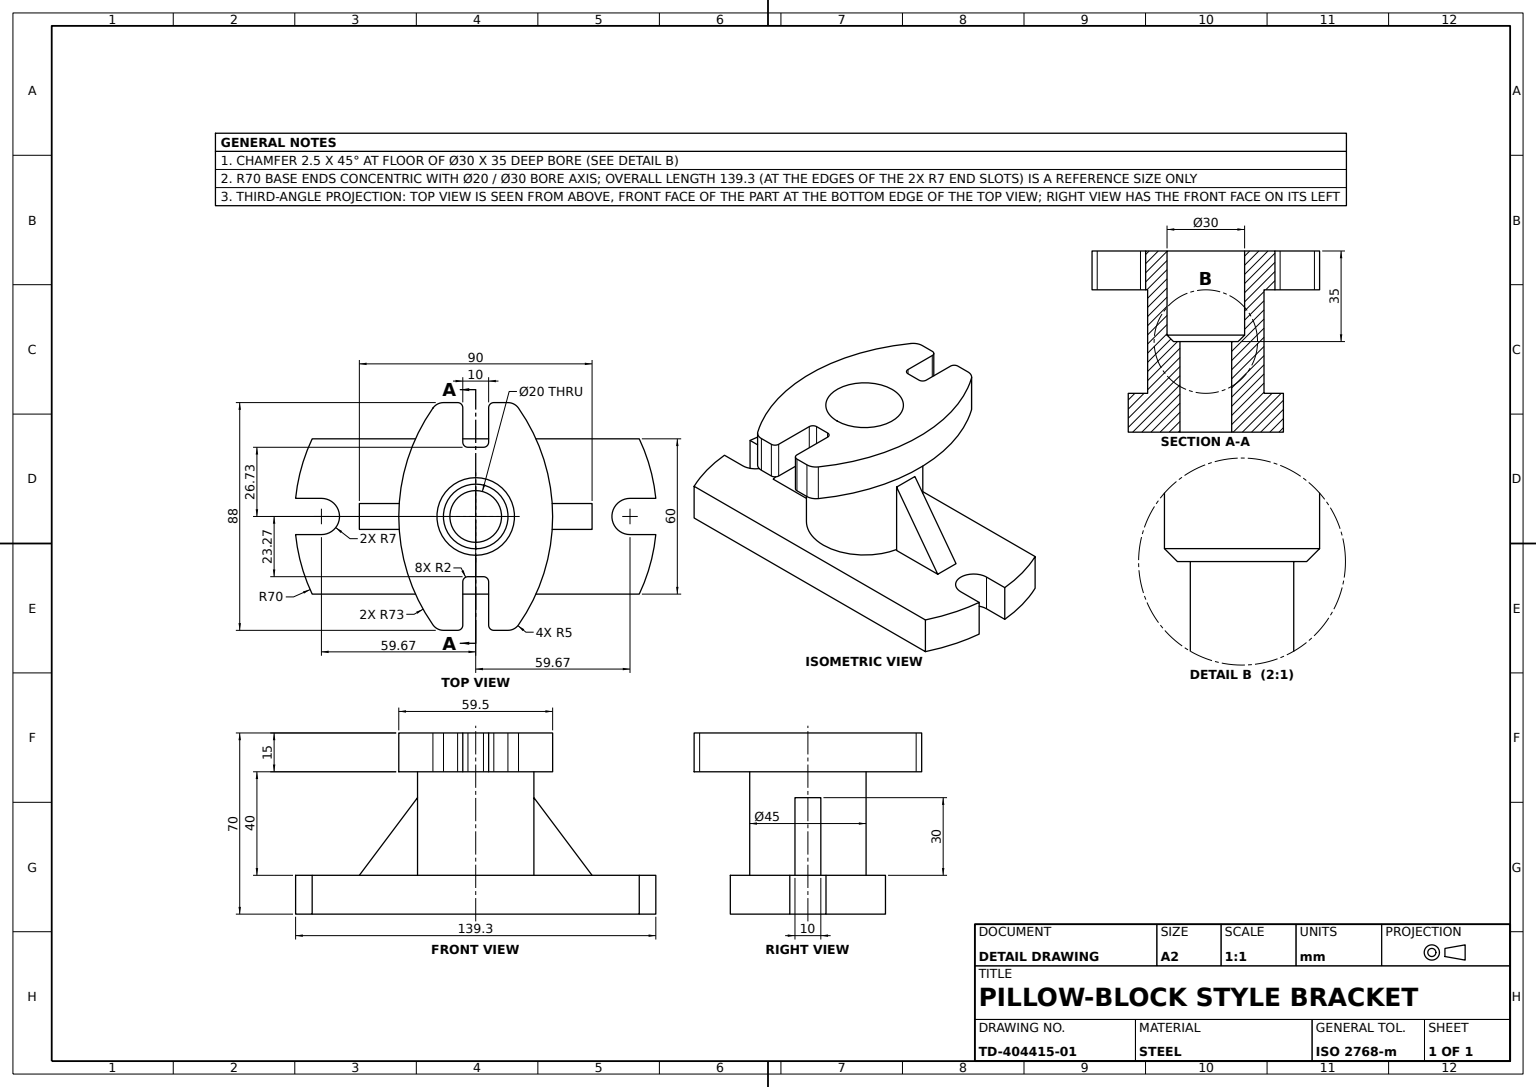
solid
v1 (22.5,45,5)
v2 (45,15,5)
e1 v1 v2 LINE
v3 (22.5,15,5)
e2 v3 v1 LINE
e3 v2 v3 LINE
face PLANE(AX(P(0,0,5),D(0,0,-1),D(1,0,0))) rev [-e1 -e2 -e3]
v4 (22.5,45,-5)
e4 v1 v4 LINE
v5 (22.5,15,-5)
e5 v5 v4 LINE
e6 v3 v5 LINE
face PLANE(AX(P(22.5,45,5),D(1,0,0),D(0,-1,0))) rev [e4 -e5 -e6 e2]
v6 (45,15,-5)
e7 v2 v6 LINE
e8 v4 v6 LINE
face PLANE(AX(P(22.5,45,5),D(-0.8,-0.6,0),D(-0.6,0.8,0))) rev [e1 e7 -e8 -e4]
e9 v6 v5 LINE
face PLANE(AX(P(45,15,5),D(0,1,0),D(0,0,1))) rev [-e9 -e7 e3 e6]
face PLANE(AX(P(0,0,-5),D(0,0,-1),D(1,0,0))) [e9 e5 e8]
solid
v7 (-22.5,15,5)
v8 (-22.5,15,-5)
e10 v7 v8 LINE
v9 (-45,15,5)
e11 v9 v7 LINE
v10 (-45,15,-5)
e12 v9 v10 LINE
e13 v10 v8 LINE
face PLANE(AX(P(-45,15,5),D(0,1,0),D(0,0,1))) rev [-e10 -e11 e12 e13]
v11 (-22.5,45,-5)
e14 v8 v11 LINE
e15 v11 v10 LINE
face PLANE(AX(P(0,0,-5),D(0,0,-1),D(-1,0,0))) [-e14 -e13 -e15]
v12 (-22.5,45,5)
e16 v12 v11 LINE
e17 v12 v9 LINE
face PLANE(AX(P(-22.5,45,5),D(0.8,-0.6,0),D(0.6,0.8,0))) rev [e16 e15 -e12 -e17]
e18 v7 v12 LINE
face PLANE(AX(P(0,0,5),D(0,0,-1),D(-1,0,0))) rev [e17 e11 e18]
face PLANE(AX(P(-22.5,45,5),D(-1,0,0),D(0,-1,0))) rev [e10 e14 -e16 -e18]
solid
v13 (0,15,-22.5)
v14 (0,15,22.5)
e19 v13 v14 CIRCLE(AX(P(0,15,0),D(0,1,0),D(0,0,1)),22.5)
e20 v14 v13 CIRCLE(AX(P(0,15,0),D(0,1,0),D(0,0,1)),22.5)
v15 (-63.245553,15,-30)
v16 (-69.649121,15,-7)
e21 v15 v16 CIRCLE(AX(P(0,15,0),D(0,1,0),D(0,0,1)),70)
v17 (-59.669311,15,-7)
e22 v16 v17 LINE
v18 (-59.669311,15,7)
e23 v17 v18 CIRCLE(AX(P(-59.669311,15,0),D(0,-1,0),D(0,0,1)),7)
v19 (-69.649121,15,7)
e24 v18 v19 LINE
v20 (-63.245553,15,30)
e25 v19 v20 CIRCLE(AX(P(0,15,0),D(0,1,0),D(0,0,1)),70)
v21 (63.245553,15,30)
e26 v20 v21 LINE
v22 (69.649121,15,7)
e27 v21 v22 CIRCLE(AX(P(0,15,0),D(0,1,0),D(0,0,1)),70)
v23 (59.669311,15,7)
e28 v22 v23 LINE
v24 (59.669311,15,-7)
e29 v23 v24 CIRCLE(AX(P(59.669311,15,0),D(0,-1,0),D(0,0,-1)),7)
v25 (69.649121,15,-7)
e30 v24 v25 LINE
v26 (63.245553,15,-30)
e31 v25 v26 CIRCLE(AX(P(0,15,0),D(0,1,0),D(0,0,1)),70)
e32 v26 v15 LINE
face PLANE(AX(P(0,15,0),D(0,1,0),D(0,0,1))) [-e19 -e20] [e21 e22 e23 e24 e25 e26 e27 e28 e29 e30 e31 e32]
v27 (-12.455114,70,44)
v28 (-12.455114,55,44)
e33 v27 v28 LINE
v29 (-7,55,44)
e34 v28 v29 LINE
v30 (-7,70,44)
e35 v30 v29 LINE
e36 v27 v30 LINE
face PLANE(AX(P(-15,70,44),D(0,0,-1),D(-1,0,0))) rev [e33 e34 -e35 -e36]
v31 (69.649121,0,7)
v32 (59.669311,0,7)
e37 v31 v32 LINE
e38 v23 v32 LINE
e39 v22 v31 LINE
face PLANE(AX(P(69.649121,15,7),D(0,0,1),D(1,0,0))) rev [e37 -e38 -e28 e39]
v33 (-5,70,42)
e40 v30 v33 CIRCLE(AX(P(-7,70,42),D(0,1,0),D(0,0,1)),2)
v34 (-5,55,42)
e41 v29 v34 CIRCLE(AX(P(-7,55,42),D(0,1,0),D(0,0,1)),2)
e42 v33 v34 LINE
face CYL(AX(P(-7,70,42),D(0,-1,0),D(0,0,-1)),2) [-e40 e35 e41 -e42]
v35 (-3,70,26.733139)
v36 (-3,55,26.733139)
e43 v35 v36 LINE
v37 (-5,70,28.733139)
e44 v37 v35 CIRCLE(AX(P(-3,70,28.733139),D(0,-1,0),D(0,0,1)),2)
v38 (-5,55,28.733139)
e45 v37 v38 LINE
e46 v38 v36 CIRCLE(AX(P(-3,55,28.733139),D(0,-1,0),D(0,0,1)),2)
face CYL(AX(P(-3,70,28.733139),D(0,-1,0),D(0,0,-1)),2) rev [-e43 -e44 e45 e46]
v39 (59.669311,0,-7)
v40 (69.649121,0,-7)
e47 v39 v40 LINE
e48 v25 v40 LINE
e49 v24 v39 LINE
face PLANE(AX(P(69.649121,15,-7),D(0,0,-1),D(-1,0,0))) rev [e47 -e48 -e30 e49]
v41 (12.455114,70,-44)
v42 (12.455114,55,-44)
e50 v41 v42 LINE
v43 (7,55,-44)
e51 v42 v43 LINE
v44 (7,70,-44)
e52 v44 v43 LINE
e53 v41 v44 LINE
face PLANE(AX(P(7,70,-44),D(0,0,1),D(1,0,0))) rev [e50 e51 -e52 -e53]
v45 (0,0,-10)
v46 (0,35,-10)
e54 v45 v46 LINE
v47 (0,0,10)
e55 v47 v45 CIRCLE(AX(P(0,0,0),D(0,1,0),D(0,0,1)),10)
v48 (0,35,10)
e56 v47 v48 LINE
e57 v48 v46 CIRCLE(AX(P(0,35,0),D(0,1,0),D(0,0,1)),10)
face CYL(AX(P(0,0,0),D(0,1,0),D(0,0,1)),10) rev [-e54 -e55 e56 e57]
e58 v32 v39 CIRCLE(AX(P(59.669311,0,0),D(0,-1,0),D(0,0,-1)),7)
face CYL(AX(P(59.669311,15,0),D(0,-1,0),D(0,0,-1)),7) rev [e58 -e49 -e29 e38]
v49 (16.551039,55,-41.867647)
v50 (16.551039,70,-41.867647)
e59 v49 v50 LINE
e60 v42 v49 CIRCLE(AX(P(12.455114,55,-39),D(0,-1,0),D(0,0,-1)),5)
e61 v50 v41 CIRCLE(AX(P(12.455114,70,-39),D(0,1,0),D(0,0,-1)),5)
face CYL(AX(P(12.455114,70,-39),D(0,-1,0),D(0,0,-1)),5) [-e59 -e60 -e50 -e61]
v51 (-69.649121,0,-7)
v52 (-59.669311,0,-7)
e62 v51 v52 LINE
e63 v17 v52 LINE
e64 v16 v51 LINE
face PLANE(AX(P(-69.649121,15,-7),D(0,0,-1),D(-1,0,0))) rev [e62 -e63 -e22 e64]
e65 v46 v48 CIRCLE(AX(P(0,35,0),D(0,1,0),D(0,0,1)),10)
e66 v45 v47 CIRCLE(AX(P(0,0,0),D(0,1,0),D(0,0,1)),10)
face CYL(AX(P(0,0,0),D(0,1,0),D(0,0,1)),10) rev [e65 -e56 -e66 e54]
v53 (7,55,44)
v54 (12.455114,55,44)
e67 v53 v54 LINE
v55 (12.455114,70,44)
e68 v54 v55 LINE
v56 (7,70,44)
e69 v56 v55 LINE
e70 v56 v53 LINE
face PLANE(AX(P(7,70,44),D(0,0,-1),D(-1,0,0))) rev [e67 e68 -e69 e70]
v57 (-7,70,-44)
v58 (-7,55,-44)
e71 v57 v58 LINE
v59 (-5,70,-42)
e72 v59 v57 CIRCLE(AX(P(-7,70,-42),D(0,1,0),D(0,0,1)),2)
v60 (-5,55,-42)
e73 v59 v60 LINE
e74 v60 v58 CIRCLE(AX(P(-7,55,-42),D(0,1,0),D(0,0,1)),2)
face CYL(AX(P(-7,70,-42),D(0,-1,0),D(0,0,-1)),2) [-e71 -e72 e73 e74]
v61 (-63.245553,0,30)
e75 v20 v61 LINE
v62 (-69.649121,0,7)
e76 v19 v62 LINE
e77 v62 v61 CIRCLE(AX(P(0,0,0),D(0,1,0),D(0,0,1)),70)
face CYL(AX(P(0,15,0),D(0,-1,0),D(0,0,-1)),70) [-e75 -e25 e76 e77]
v63 (0,70,-15)
v64 (0,70,15)
e78 v63 v64 CIRCLE(AX(P(0,70,0),D(0,1,0),D(0,0,1)),15)
e79 v64 v63 CIRCLE(AX(P(0,70,0),D(0,1,0),D(0,0,1)),15)
v65 (16.551039,70,41.867647)
e80 v55 v65 CIRCLE(AX(P(12.455114,70,39),D(0,1,0),D(0,0,-1)),5)
e81 v65 v50 CIRCLE(AX(P(-43.249464,70,0),D(0,1,0),D(0,0,-1)),73)
v66 (5,70,-42)
e82 v44 v66 CIRCLE(AX(P(7,70,-42),D(0,1,0),D(0,0,-1)),2)
v67 (5,70,-25.266861)
e83 v66 v67 LINE
v68 (3,70,-23.266861)
e84 v67 v68 CIRCLE(AX(P(3,70,-25.266861),D(0,-1,0),D(0,0,1)),2)
v69 (-3,70,-23.266861)
e85 v68 v69 LINE
v70 (-5,70,-25.266861)
e86 v69 v70 CIRCLE(AX(P(-3,70,-25.266861),D(0,-1,0),D(0,0,-1)),2)
e87 v70 v59 LINE
v71 (-12.455114,70,-44)
e88 v57 v71 LINE
v72 (-16.551039,70,-41.867647)
e89 v71 v72 CIRCLE(AX(P(-12.455114,70,-39),D(0,1,0),D(0,0,-1)),5)
v73 (-16.551039,70,41.867647)
e90 v72 v73 CIRCLE(AX(P(43.249464,70,0),D(0,1,0),D(0,0,1)),73)
e91 v73 v27 CIRCLE(AX(P(-12.455114,70,39),D(0,1,0),D(0,0,-1)),5)
e92 v33 v37 LINE
v74 (3,70,26.733139)
e93 v35 v74 LINE
v75 (5,70,28.733139)
e94 v74 v75 CIRCLE(AX(P(3,70,28.733139),D(0,-1,0),D(0,0,-1)),2)
v76 (5,70,42)
e95 v75 v76 LINE
e96 v76 v56 CIRCLE(AX(P(7,70,42),D(0,1,0),D(0,0,1)),2)
face PLANE(AX(P(-43.249464,70,0),D(0,-1,0),D(0,0,-1))) rev [-e78 -e79] [e69 e80 e81 e61 e53 e82 e83 e84 e85 e86 e87 e72 e88 e89 e90 e91 e36 e40 e92 e44 e93 e94 e95 e96]
v77 (5,55,42)
e97 v76 v77 LINE
e98 v77 v53 CIRCLE(AX(P(7,55,42),D(0,1,0),D(0,0,1)),2)
face CYL(AX(P(7,70,42),D(0,-1,0),D(0,0,-1)),2) [-e96 e97 e98 -e70]
v78 (-16.551039,55,-41.867647)
e99 v72 v78 LINE
v79 (-16.551039,55,41.867647)
e100 v78 v79 CIRCLE(AX(P(43.249464,55,0),D(0,1,0),D(0,0,1)),73)
e101 v79 v73 LINE
face CYL(AX(P(43.249464,70,0),D(0,-1,0),D(0,0,-1)),73) [-e90 e99 e100 e101]
e102 v34 v38 LINE
face PLANE(AX(P(-5,70,42),D(-1,0,0),D(0,0,1))) rev [-e45 -e92 e42 e102]
v80 (5,55,-42)
e103 v66 v80 LINE
v81 (5,55,-25.266861)
e104 v80 v81 LINE
e105 v67 v81 LINE
face PLANE(AX(P(5,70,-42),D(1,0,0),D(0,0,-1))) rev [-e83 e103 e104 -e105]
v82 (0,35,-12.5)
v83 (0,35,12.5)
e106 v82 v83 CIRCLE(AX(P(0,35,0),D(0,1,0),D(0,0,1)),12.5)
v84 (0,37.5,-15)
e107 v82 v84 LINE
v85 (0,37.5,15)
e108 v85 v84 CIRCLE(AX(P(0,37.5,0),D(0,-1,0),D(0,0,1)),15)
e109 v83 v85 LINE
face CONE(AX(P(0,35,0),D(0,1,0),D(0,0,1)),12.5,0.785398163) rev [-e106 e107 -e108 -e109]
v86 (-5,55,-25.266861)
e110 v70 v86 LINE
v87 (-3,55,-23.266861)
e111 v69 v87 LINE
e112 v87 v86 CIRCLE(AX(P(-3,55,-25.266861),D(0,-1,0),D(0,0,-1)),2)
face CYL(AX(P(-3,70,-25.266861),D(0,-1,0),D(0,0,-1)),2) rev [-e110 -e86 e111 e112]
v88 (-12.455114,55,-44)
e113 v88 v71 LINE
e114 v78 v88 CIRCLE(AX(P(-12.455114,55,-39),D(0,-1,0),D(0,0,-1)),5)
face CYL(AX(P(-12.455114,70,-39),D(0,-1,0),D(0,0,-1)),5) [-e99 -e89 -e113 -e114]
e115 v83 v82 CIRCLE(AX(P(0,35,0),D(0,1,0),D(0,0,1)),12.5)
face PLANE(AX(P(0,35,0),D(0,1,0),D(0,0,1))) [e115 e106] [-e65 -e57]
v89 (63.245553,0,-30)
e116 v26 v89 LINE
e117 v40 v89 CIRCLE(AX(P(0,0,0),D(0,1,0),D(0,0,1)),70)
face CYL(AX(P(0,15,0),D(0,-1,0),D(0,0,-1)),70) [-e116 -e31 e48 e117]
v90 (16.551039,55,41.867647)
e118 v90 v54 CIRCLE(AX(P(12.455114,55,39),D(0,-1,0),D(0,0,-1)),5)
e119 v65 v90 LINE
face CYL(AX(P(12.455114,70,39),D(0,-1,0),D(0,0,-1)),5) [-e68 -e118 -e119 -e80]
v91 (3,55,-23.266861)
e120 v91 v87 LINE
e121 v68 v91 LINE
face PLANE(AX(P(-3,70,-23.266861),D(0,0,1),D(1,0,0))) rev [e120 -e111 -e85 e121]
e122 v85 v64 LINE
e123 v84 v63 LINE
face CYL(AX(P(0,35,0),D(0,1,0),D(0,0,1)),15) rev [e78 -e122 e108 e123]
e124 v86 v60 LINE
face PLANE(AX(P(-5,70,-42),D(-1,0,0),D(0,0,1))) rev [e110 e124 -e73 -e87]
v92 (0,55,22.5)
v93 (0,55,-22.5)
e125 v92 v93 CIRCLE(AX(P(0,55,0),D(0,1,0),D(0,0,1)),22.5)
e126 v92 v14 LINE
e127 v93 v13 LINE
face CYL(AX(P(0,55,0),D(0,-1,0),D(0,0,-1)),22.5) [-e125 e126 e20 -e127]
e128 v81 v91 CIRCLE(AX(P(3,55,-25.266861),D(0,-1,0),D(0,0,1)),2)
face CYL(AX(P(3,70,-25.266861),D(0,-1,0),D(0,0,-1)),2) rev [-e121 -e84 e105 e128]
v94 (63.245553,0,30)
e129 v61 v94 LINE
e130 v21 v94 LINE
face PLANE(AX(P(-63.245553,15,30),D(0,0,-1),D(-1,0,0))) rev [e75 e129 -e130 -e26]
e131 v58 v88 LINE
face PLANE(AX(P(-15,70,-44),D(0,0,1),D(1,0,0))) rev [e71 e131 e113 -e88]
v95 (3,55,26.733139)
e132 v36 v95 LINE
e133 v74 v95 LINE
face PLANE(AX(P(-3,70,26.733139),D(0,0,-1),D(-1,0,0))) rev [-e93 e43 e132 -e133]
e134 v28 v79 CIRCLE(AX(P(-12.455114,55,39),D(0,-1,0),D(0,0,-1)),5)
face CYL(AX(P(-12.455114,70,39),D(0,-1,0),D(0,0,-1)),5) [-e134 -e33 -e91 -e101]
v96 (-63.245553,0,-30)
e135 v89 v96 LINE
e136 v15 v96 LINE
face PLANE(AX(P(-63.245553,15,-30),D(0,0,1),D(1,0,0))) rev [e135 -e136 -e32 e116]
v97 (-59.669311,0,7)
e137 v52 v97 CIRCLE(AX(P(-59.669311,0,0),D(0,-1,0),D(0,0,1)),7)
e138 v18 v97 LINE
face CYL(AX(P(-59.669311,15,0),D(0,-1,0),D(0,0,-1)),7) rev [e63 e137 -e138 -e23]
v98 (5,55,28.733139)
e139 v95 v98 CIRCLE(AX(P(3,55,28.733139),D(0,-1,0),D(0,0,-1)),2)
e140 v75 v98 LINE
face CYL(AX(P(3,70,28.733139),D(0,-1,0),D(0,0,-1)),2) rev [e133 e139 -e140 -e94]
e141 v94 v31 CIRCLE(AX(P(0,0,0),D(0,1,0),D(0,0,1)),70)
face CYL(AX(P(0,15,0),D(0,-1,0),D(0,0,-1)),70) [-e27 e130 e141 -e39]
e142 v93 v92 CIRCLE(AX(P(0,55,0),D(0,1,0),D(0,0,1)),22.5)
face CYL(AX(P(0,55,0),D(0,-1,0),D(0,0,-1)),22.5) [e19 -e126 -e142 e127]
e143 v96 v51 CIRCLE(AX(P(0,0,0),D(0,1,0),D(0,0,1)),70)
face CYL(AX(P(0,15,0),D(0,-1,0),D(0,0,-1)),70) [e136 e143 -e64 -e21]
e144 v84 v85 CIRCLE(AX(P(0,37.5,0),D(0,-1,0),D(0,0,1)),15)
face CYL(AX(P(0,35,0),D(0,1,0),D(0,0,1)),15) rev [e122 e79 -e123 e144]
e145 v43 v80 CIRCLE(AX(P(7,55,-42),D(0,1,0),D(0,0,-1)),2)
face CYL(AX(P(7,70,-42),D(0,-1,0),D(0,0,-1)),2) [-e82 e52 e145 -e103]
e146 v90 v49 CIRCLE(AX(P(-43.249464,55,0),D(0,1,0),D(0,0,-1)),73)
e147 v98 v77 LINE
face PLANE(AX(P(-43.249464,55,0),D(0,-1,0),D(0,0,-1))) [e142 e125] [-e51 e60 -e146 e118 -e67 -e98 -e147 -e139 -e132 -e46 -e102 -e41 -e34 e134 -e100 e114 -e131 -e74 -e124 -e112 -e120 -e128 -e104 -e145]
e148 v97 v62 LINE
face PLANE(AX(P(-69.649121,15,7),D(0,0,1),D(1,0,0))) rev [-e76 -e24 e138 e148]
face CONE(AX(P(0,35,0),D(0,1,0),D(0,0,1)),12.5,0.785398163) rev [e109 -e144 -e107 -e115]
face CYL(AX(P(-43.249464,70,0),D(0,-1,0),D(0,0,-1)),73) [e119 e146 e59 -e81]
face PLANE(AX(P(0,0,0),D(0,1,0),D(0,0,1))) rev [e55 e66] [-e143 -e135 -e117 -e47 -e58 -e37 -e141 -e129 -e77 -e148 -e137 -e62]
face PLANE(AX(P(5,70,42),D(1,0,0),D(0,0,-1))) rev [e147 -e97 -e95 e140]
